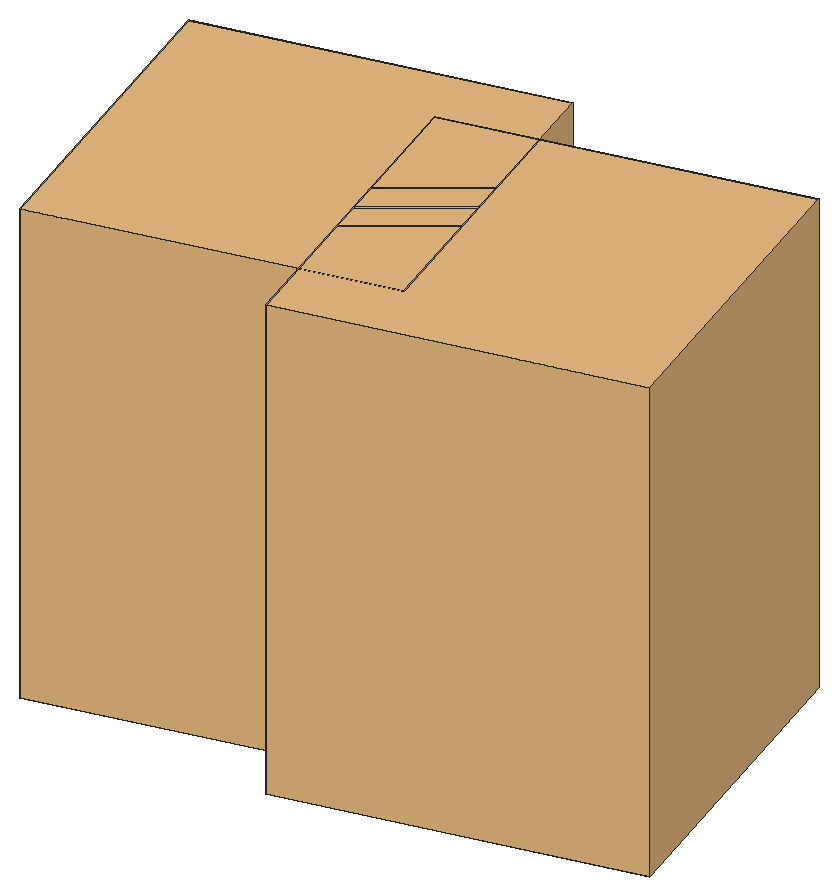
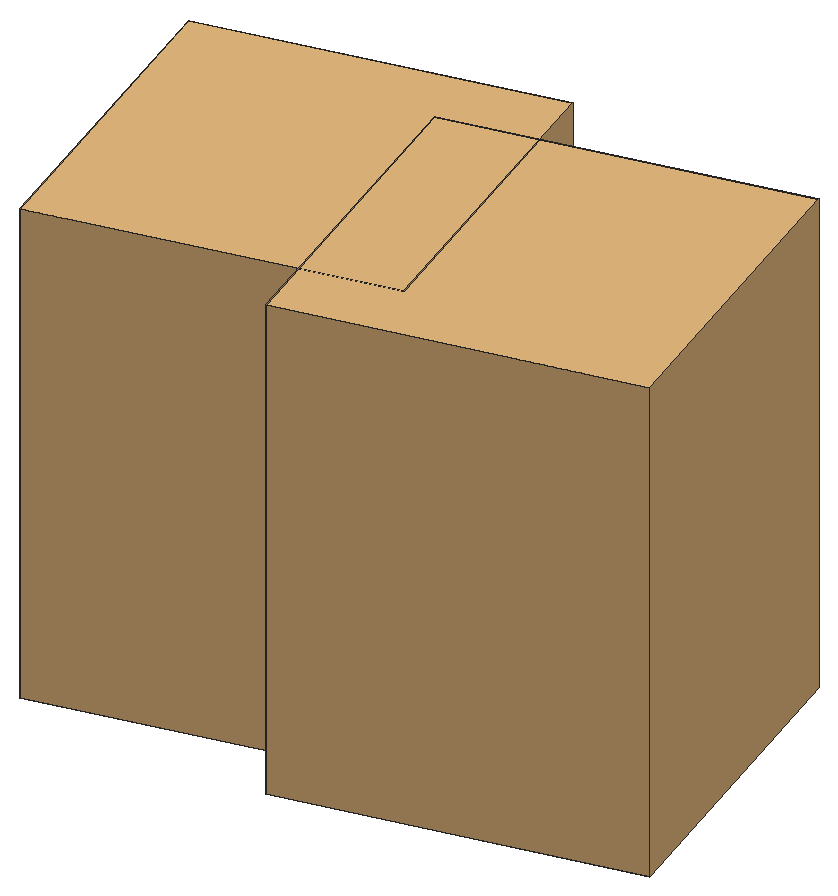
# SketchUp Ruby script. Lengths in inches.
U = 1.inch
M = Sketchup.active_model
def pt(a) = Geom::Point3d.new(a.map { |v| v * U })
def face(e, loops, mat)
  f = e.add_face(loops[0].map { |a| pt(a) })
  loops[1..].each { |l| e.add_face(l.map { |a| pt(a) }).erase! }
  f.material = f.back_material = mat if mat
  f
end
# faces: each face lists its corners as indices into pts; further lists are holes
def faces(e, pts, list, mat = nil) = list.each { |f| face(e, (f[0].is_a?(Array) ? f : [f]).map { |l| l.map { |i| pts[i] } }, mat) }
# xy, xz, yz: faces in a plane at the given z, y or x. An outline is a flat list of corners, or four numbers for a rectangle; further outlines are holes
def ring(l) = l.size == 4 ? [[l[0], l[1]], [l[2], l[1]], [l[2], l[3]], [l[0], l[3]]] : l.each_slice(2).to_a
def flat(e, list, mat, &to3) = list.each { |f| face(e, (f[0].is_a?(Array) ? f : [f]).map { |l| ring(l).map { |u, v| to3.(u, v) } }, mat) }
def xy(e, z, list, mat = nil) = flat(e, list, mat) { |x, y| [x, y, z] }
def xz(e, y, list, mat = nil) = flat(e, list, mat) { |x, z| [x, y, z] }
def yz(e, x, list, mat = nil) = flat(e, list, mat) { |y, z| [x, y, z] }
def lines(e, pts, list) = list.each { |a, b| e.add_line(pt(pts[a]), pt(pts[b])) }
# prism: a flat outline (further loops are holes) pulled along v
def prism(e, loops, v, mat = nil)
  f = face(e, loops, mat); d = Geom::Vector3d.new(v.map { |x| x * U })
  f.pushpull(f.normal.samedirection?(d) ? d.length : -d.length)
end
def box(e, o, s, mat = nil) = prism(e, [[o, [o[0] + s[0], o[1], o[2]], [o[0] + s[0], o[1] + s[1], o[2]], [o[0], o[1] + s[1], o[2]]]], [0, 0, s[2]], mat)
def at(x, y, z, deg = 0) = Geom::Transformation.translation(pt([x, y, z])) * Geom::Transformation.rotation(ORIGIN, Z_AXIS, deg.degrees)
def axes(o, x, y, z) = Geom::Transformation.new([*x, 0, *y, 0, *z, 0, *pt(o).to_a, 1])
def part(name) = M.definitions.add(name)
# library, detail: a bought-in or finely detailed component or shape, given as its bounding box
def library(name, o, s) = part(name).tap { |d| box(d.entities, o, s) }
def detail(e, o, s) = box(e.add_group.entities, o, s)
def put(e, d, t, mat = nil) = e.add_instance(d, t).tap { |i| i.material = mat if mat }
def group(e, t, mat = nil) = e.add_group.tap { |g| g.transformation = t; g.material = mat if mat }.entities
root = M.entities
M.materials.add("Material82").color = [68, 110, 58]
M.materials.add("Material83").color = [48, 90, 38]
M.materials.add("Material84").color = [68, 110, 48]
M.materials.add("Material85").color = [48, 90, 48]
M.materials.add("Material86").color = [58, 110, 58]
M.materials.add("Material87").color = [58, 90, 38]
M.materials.add("Material88").color = [68, 100, 58]
M.materials.add("Material89").color = [48, 100, 38]
c1 = part("grass00")
p = [[-0.6875,0.15,0],[-0.56,0.08,5.52],[-0.04,0.03,2.76],[0.48,-0.02,0],[0.35,-0.02,5.52],[-0.1,-0.14,5.52],
  [-0.12,0.65,8.37],[-0.42,0.65,8.37]]
faces(c1.entities,p,[[0,1,2,3],[3,2,4],[1,5,2],[5,4,2],[1,6,5],[4,5,6],[7,6,1]])
c2 = part("Group16\#1")
put(c2.entities,c1,axes([1.44,-0.61,-0.01],[0.05352,0.12609,0],[-0.10704,0.04543,0.07239],[0.06664,-0.02828,0.11628]),"Material85")
put(c2.entities,c1,axes([0.76,-0.15,-0.01],[0.04676,0.24062,0],[-0.23162,0.04501,0.06642],[0.0652,-0.01267,0.23595]),"Material82")
put(c2.entities,c1,axes([0.79,0.01,-0.01],[-0.00606,0.34651,0],[-0.34381,-0.00602,0.0432],[0.04319,0.00076,0.34386]))
put(c2.entities,c1,axes([1,0.23,-0.01],[-0.07192,0.31144,0],[-0.28722,-0.06632,0.1236],[0.12043,0.02781,0.29478]),"Material84")
put(c2.entities,c1,axes([1.66,0.77,-0.01],[-0.13828,0.29651,0],[-0.21551,-0.1005,0.22471],[0.20365,0.09498,0.23779]),"Material89")
put(c2.entities,c1,axes([0.6875,0.52,-0.01],[-0.18126,0.24051,0],[-0.22746,-0.17142,0.09788],[0.07817,0.05891,0.28481]),"Material84")
put(c2.entities,c1,axes([0.68,0.78,-0.01],[-0.215,0.18688,0],[-0.12385,-0.14248,0.21334],[0.13995,0.16101,0.18878]),"Material82")
put(c2.entities,c1,axes([0.56,1,-0.01],[-0.13756,0.07624,0],[-0.06159,-0.11112,0.0927],[0.04494,0.08108,0.12705]),"Material84")
put(c2.entities,c1,axes([0.2,0.64,-0.01],[-0.23729,0.07254,0],[-0.05711,-0.18681,0.153],[0.04473,0.14632,0.19535]),"Material89")
put(c2.entities,c1,axes([0.0625,0.72,-0.01],[-0.28874,0.02525,0],[-0.02179,-0.24916,0.14647],[0.01276,0.14591,0.25012]),"Material82")
put(c2.entities,c1,axes([-0.08,0.62,-0.01],[-0.34089,-0.04187,0],[0.03255,-0.26504,0.216],[-0.02633,0.21439,0.26703]),"Material89")
put(c2.entities,c1,axes([-0.34,0.98,-0.01],[-0.14314,-0.0493,0],[0.04397,-0.12769,0.06843],[-0.02228,0.0647,0.13505]),"Material89")
put(c2.entities,c1,axes([-0.87,1.45,-0.01],[-0.23488,-0.14114,0],[0.13761,-0.22901,0.06087],[-0.03135,0.05217,0.26717]))
put(c2.entities,c1,axes([-0.72,0.77,-0.01],[-0.14208,-0.13251,0],[0.07209,-0.0773,0.16301],[-0.11118,0.11922,0.1057]),"Material89")
put(c2.entities,c1,axes([-0.62,0.43,-0.01],[-0.14845,-0.21203,0],[0.18654,-0.13061,0.12304],[-0.10079,0.07057,0.22772]),"Material82")
put(c2.entities,c1,axes([-0.68,0.29,-0.01],[-0.13639,-0.32136,0],[0.31723,-0.13464,0.05579],[-0.05136,0.0218,0.34462]),"Material83")
put(c2.entities,c1,axes([-0.64,0.125,-0.01],[-0.0458,-0.23569,0],[0.22124,-0.043,0.08276],[-0.08124,0.01579,0.22538]),"Material86")
put(c2.entities,c1,axes([-1.6,-0.03,-0.01],[0.00576,-0.32897,0],[0.27526,0.00482,0.18018],[-0.18015,-0.00315,0.2753]),"Material84")
put(c2.entities,c1,axes([-1.36,-0.31,-0.01],[0.05718,-0.24765,0],[0.18172,0.04196,0.17267],[-0.16825,-0.03885,0.1865]),"Material89")
put(c2.entities,c1,axes([-1.54,-0.72,-0.01],[0.06537,-0.14017,0],[0.13555,0.06321,0.03939],[-0.0357,-0.01665,0.14956]))
put(c2.entities,c1,axes([-1.19,-0.9,-0.01],[0.09597,-0.12735,0],[0.11214,0.08451,0.07557],[-0.06035,-0.04548,0.14042]),"Material88")
put(c2.entities,c1,axes([-0.47,-0.54,-0.01],[0.11588,-0.10072,0],[0.0618,0.0711,0.12124],[-0.07953,-0.0915,0.0942]))
put(c2.entities,c1,axes([-0.47,-0.84,-0.01],[0.11927,-0.0661,0],[0.06603,0.11913,0.00646],[-0.00313,-0.00565,0.13621]),"Material84")
put(c2.entities,c1,axes([-0.38,-1.24,-0.01],[0.28037,-0.08571,0],[0.0618,0.20215,0.20315],[-0.05939,-0.19428,0.21139]),"Material88")
put(c2.entities,c1,axes([-0.06,-0.66,-0.01],[0.22719,-0.01987,0],[0.01247,0.14255,0.17758],[-0.01547,-0.17691,0.1431]),"Material87")
put(c2.entities,c1,axes([0.11,-0.89,-0.01],[0.14882,0.01828,0],[-0.01058,0.08611,0.12229],[0.01491,-0.12138,0.08676]),"Material85")
put(c2.entities,c1,axes([0.25,-0.72,-0.01],[0.20481,0.07053,0],[-0.06206,0.18022,0.10291],[0.03351,-0.0973,0.1906]),"Material85")
put(c2.entities,c1,axes([0.85,-1.42,-0.01],[0.16481,0.09904,0],[-0.09472,0.15762,0.05616],[0.02893,-0.04814,0.18389]),"Material84")
put(c2.entities,c1,axes([1.01,-1.09,-0.01],[0.21858,0.20385,0],[-0.17495,0.1876,0.15339],[0.10462,-0.11218,0.25652]),"Material89")
put(c2.entities,c1,axes([1.01,-0.71,-0.01],[0.08733,0.12473,0],[-0.06445,0.04512,0.13037],[0.1068,-0.07477,0.07867]),"Material85")
c3 = part("Group15\#1")
put(c3.entities,c2,at(0,0,0))
c4 = part("3darcstudiotree_grass00\#1")
put(c4.entities,c3,at(0,0,0))
c5 = library("Palm tree",[-4.09,-4.52,0],[193.52,193.51,258.93])
c6 = part("Palm+Tree")
put(c6.entities,c5,at(25.51,-21.81,0,15))
c7 = library("Group\#612",[0,0,0],[32.91,53.52,103.45])
put(root,c4,axes([1856.3125,966.58,-29.74],[3.38368,1.04745,0],[-2.27938,1.14521,-0.02005],[-0.08327,0.04184,1.86077]))
put(root,c4,axes([1858.36,994.28,-29.74],[0.01113,-1.45353,0],[4.54919,0.00542,-0.03692],[0.17089,0.0002,1.57831]))
put(root,c4,axes([1858.7,972.38,-29.74],[-1.2969,-1.20265,0],[3.80092,-0.63749,-0.01791],[0.10113,-0.01696,1.89984]))
put(root,c4,axes([1858.8,950.74,-29.74],[0.25593,-1.38573,0],[3.33259,0.09573,-0.00937],[0.07232,0.00208,1.93766]))
put(root,c4,axes([1858.69,946.16,-29.74],[-3.13946,0.49629,0],[-1.50487,-1.48058,-0.04281],[-0.09532,-0.09378,1.81418]))
put(root,c4,axes([1858.58,988.9,-29.74],[3.11316,-1.08854,0],[2.76667,1.23063,-0.03392],[0.0954,0.04244,1.32537]))
put(root,c4,axes([1859.6875,957.3,-29.74],[-3.90762,0.14516,0],[-0.37668,-1.57704,-0.0202],[-0.01231,-0.05153,1.95637]))
put(root,c4,axes([1858.54,941.52,-29.74],[3.63772,-0.04618,0],[0.1059,1.29755,-0.04101],[0.00733,0.08987,1.37186]))
put(root,c4,axes([1858.61,996.94,-29.74],[0.13497,1.53866,0],[-3.75353,0.05121,-0.02489],[-0.17047,0.00233,1.9295]))
put(root,c4,axes([1859.17,992.46,-29.74],[-2.50392,0.92561,0],[-3.00944,-1.26617,-0.02311],[-0.06646,-0.02796,1.38694]))
put(root,c4,axes([1860.33,985.73,-29.74],[-4.13167,0.24366,0],[-0.69238,-1.82599,-0.06496],[-0.05165,-0.1362,1.88637]))
put(root,c4,axes([1859.52,968.625,-29.74],[-1.70819,1.11812,0],[-3.96876,-0.943,-0.04504],[-0.21667,-0.05148,1.9506]))
put(root,c4,axes([1859.7,977.74,-29.74],[3.79912,-1.05543,0],[2.19489,1.22878,-0.03692],[0.13668,0.07652,1.83631]))
put(root,c4,axes([1859.58,943.99,-29.74],[3.28657,0.21022,0],[-0.53923,1.31117,-0.01255],[-0.01302,0.03166,1.63564]))
put(root,c4,axes([1860.18,983.93,-29.74],[-2.37455,1.29783,0],[-2.73236,-0.77752,-0.00844],[-0.03827,-0.01089,1.41311]))
put(root,c4,axes([1859.5,974.99,-29.74],[2.3712,1.21069,0],[-3.58151,1.09097,-0.04605],[-0.15475,0.04714,1.44046]))
put(root,c4,axes([1860.73,960.11,-29.74],[1.66455,-1.14728,0],[3.31311,0.74761,-0.04415],[0.26641,0.06012,1.98924]))
put(root,c4,axes([1861.84,990.33,-29.74],[-0.63027,-1.58552,0],[4.65732,-0.28794,-0.06318],[0.24644,-0.01524,1.39517]))
put(root,c4,axes([1860.29,961.55,-29.74],[2.52471,1.58546,0],[-3.52346,0.87265,-0.052],[-0.25077,0.06211,1.7759]))
put(root,c4,axes([1861.07,982.34,-29.74],[3.33412,-1.28398,0],[2.96352,1.19685,-0.04175],[0.14903,0.06019,1.62422]))
put(root,c4,axes([1860.47,978.86,-29.74],[3.98735,0.11869,0],[-0.3473,1.81468,-0.00004],[-0.00002,0.00009,1.93334]))
put(root,c4,axes([1862.11,953.3125,-29.74],[-2.08457,-1.53905,0],[3.84719,-0.81044,-0.05822],[0.30315,-0.06386,1.92982]))
put(root,c4,axes([1861.24,970.21,-29.74],[0.24653,1.78059,0],[-4.18646,0.09015,-0.05861],[-0.36644,0.00789,1.96776]))
put(root,c4,axes([1860.75,964.86,-29.74],[4.09909,0.70116,0],[-1.55013,1.40946,-0.01845],[-0.03388,0.03081,1.34771]))
put(root,c4,axes([1860.79,940.48,-29.74],[1.95248,1.61036,0],[-3.842,0.72449,-0.01048],[-0.04175,0.00787,1.40926]))
put(root,c4,axes([1861.11,955.24,-29.74],[3.93599,0.37319,0],[-1.10472,1.81211,-0.03506],[-0.03066,0.05029,1.32515]))
put(root,c4,axes([1861.76,948.9,-29.74],[3.76504,-0.34797,0],[1.07827,1.81452,-0.02268],[0.0226,0.03802,1.5468]))
put(root,c4,axes([1861.75,965.91,-29.74],[-0.03028,1.81071,0],[-4.52004,-0.01176,-0.01347],[-0.05788,-0.00015,1.45625]))
put(root,c4,axes([1863.97,947.37,-29.74],[2.88127,-0.83898,0],[2.47269,1.32072,-0.02283],[0.06307,0.03369,1.4512]))
put(root,c4,axes([1864.89,952.36,-29.74],[-1.69688,-1.72936,0],[4.23511,-0.64631,-0.05475],[0.2829,-0.04317,1.88574]))
put(root,c4,axes([1863.97,944.48,-29.74],[3.22121,-0.88629,0],[2.07064,1.17047,-0.00731],[0.02777,0.0157,1.80073]))
put(root,c4,axes([1865.1,994.51,-29.74],[-1.90792,-1.42621,0],[3.47826,-0.72369,-0.03938],[0.16408,-0.03414,1.38871]))
put(root,c4,axes([1864.16,981.1,-29.74],[3.56261,-0.94567,0],[1.87037,1.0959,-0.0013],[0.00431,0.00253,1.49257]))
put(root,c4,axes([1864.0625,955.86,-29.74],[-1.05565,1.36177,0],[-3.91341,-0.47183,-0.0271],[-0.14616,-0.01762,1.72974]))
put(root,c4,axes([1865.36,948.53,-29.74],[-4.0685,0.50795,0],[-1.17773,-1.46714,-0.03323],[-0.06082,-0.07576,1.77353]))
put(root,c4,axes([1864.42,941.89,-29.74],[4.25936,0.17724,0],[-0.36955,1.38123,-0.03171],[-0.02162,0.08082,1.71518]))
put(root,c4,axes([1866.03,958.15,-29.74],[0.20903,-1.7077,0],[3.89534,0.07416,-0.00402],[0.01821,0.00035,1.3243]))
put(root,c4,axes([1866.13,964.27,-29.74],[-3.49989,-0.62042,0],[1.34924,-1.18377,-0.02079],[0.0557,-0.04887,1.61237]))
put(root,c4,axes([1865.39,966.43,-29.74],[-2.24971,1.27376,0],[-2.901,-0.79689,-0.01437],[-0.08541,-0.02346,1.91898]))
put(root,c4,axes([1866.29,988.83,-29.74],[-2.13915,-1.27276,0],[3.26215,-0.85272,-0.05028],[0.27845,-0.07279,1.94898]))
put(root,c4,axes([1865.16,992.79,-29.74],[4.02195,-0.32221,0],[0.68718,1.33408,-0.00331],[0.00405,0.00786,1.58887]))
put(root,c4,axes([1864.66,979.09,-29.74],[4.32701,0.55712,0],[-1.36775,1.65217,-0.00124],[-0.00192,0.00232,1.65228]))
put(root,c4,axes([1865.85,986.48,-29.74],[-1.63539,1.16071,0],[-3.40916,-0.74706,-0.05151],[-0.29339,-0.06429,1.90487]))
put(root,c4,axes([1865.06,983.57,-29.74],[1.01762,1.37596,0],[-4.26505,0.49058,-0.00405],[-0.01582,0.00182,1.35389]))
put(root,c4,axes([1867.35,975.45,-29.74],[-3.3697,-1.02042,0],[2.44227,-1.25434,-0.00705],[0.02625,-0.01348,1.8369]))
put(root,c4,axes([1866.49,977.03,-29.74],[2.02024,-1.18426,0],[3.76291,0.99837,-0.06298],[0.20491,0.05437,1.33293]))
put(root,c4,axes([1865.71,940.4,-29.74],[4.3094,-0.16311,0],[0.42718,1.75528,-0.01064],[0.00539,0.02213,1.77558]))
put(root,c4,axes([1867.47,990.66,-29.74],[-2.95002,-1.42448,0],[3.56758,-1.14909,-0.03335],[0.13906,-0.04479,1.85855]))
put(root,c4,axes([1866.9,971.42,-29.74],[0.35372,-1.85816,0],[4.64402,0.13749,-0.06273],[0.35272,0.01044,1.9684]))
put(root,c4,axes([1866.49,950.38,-29.74],[-1.74852,1.13217,0],[-3.21789,-0.77293,-0.03041],[-0.12145,-0.02917,1.3205]))
put(root,c4,axes([1867.8125,969.18,-29.74],[-1.80602,-1.23313,0],[3.1704,-0.72217,-0.00817],[0.04009,-0.00913,1.55447]))
put(root,c4,axes([1867.05,972.1,-29.74],[3.72507,-0.62439,0],[1.73357,1.60854,-0.00549],[0.00931,0.00864,1.44062]))
put(root,c4,axes([1867.05,960.3,-29.74],[3.99736,-0.43263,0],[1.22188,1.75587,-0.05143],[0.05673,0.08152,1.44218]))
put(root,c4,axes([1867.01,962.125,-29.74],[-0.70731,1.48216,0],[-4.42453,-0.32839,-0.01956],[-0.1033,-0.00767,1.8138]))
put(root,c4,axes([1869.49,958,-29.74],[-4.33089,0.41445,0],[-1.11243,-1.80796,-0.06662],[-0.06204,-0.10083,1.39642]))
put(root,c4,axes([1870.375,948.14,-29.74],[-3.26976,-0.5137,0],[1.67175,-1.65498,-0.00121],[0.00254,-0.00252,1.92636]))
put(root,c4,axes([1869.61,992.46,-29.74],[1.4091,-1.17417,0],[3.00858,0.56155,-0.04441],[0.31581,0.05895,1.96303]))
put(root,c4,axes([1870.35,988.18,-29.74],[-0.33318,-1.39627,0],[3.47077,-0.12881,-0.04952],[0.2452,-0.0091,1.29958]))
put(root,c4,axes([1870.46,983.83,-29.74],[-3.53744,1.16554,0],[-2.5606,-1.20869,-0.03098],[-0.10582,-0.04995,1.59479]))
put(root,c4,axes([1871.08,996.27,-29.74],[-3.84526,-0.22431,0],[0.50015,-1.33348,-0.00812],[0.00644,-0.01718,1.3892]))
put(root,c4,axes([1870.6,978.95,-29.74],[-3.00421,0.76942,0],[-2.15411,-1.30812,-0.04277],[-0.14646,-0.08894,1.86401]))
put(root,c4,axes([1870.06,950.6,-29.74],[-0.58592,1.57945,0],[-3.44253,-0.19862,-0.02144],[-0.15876,-0.00916,1.9513]))
put(root,c4,axes([1870.57,971.43,-29.74],[-3.04736,0.88871,0],[-2.40783,-1.28411,-0.01371],[-0.03527,-0.01881,1.31321]))
put(root,c4,axes([1870.0625,990.875,-29.74],[3.34176,-0.01383,0],[0.04057,1.52455,-0.01029],[0.00052,0.01945,1.389]))
put(root,c4,axes([1871.1875,955.2,-29.74],[1.49416,-1.17809,0],[3.55261,0.70077,-0.01805],[0.08589,0.01694,1.58457]))
put(root,c4,axes([1870.31,977.41,-29.74],[3.91979,-0.74164,0],[1.60866,1.32236,-0.04597],[0.11253,0.0925,1.57738]))
put(root,c4,axes([1870.49,974.67,-29.74],[-2.1963,1.32957,0],[-3.96988,-1.01993,-0.00953],[-0.0332,-0.00853,1.47621]))
put(root,c4,axes([1871.74,994.88,-29.74],[0.96851,-1.36822,0],[3.89034,0.4283,-0.00232],[0.01298,0.00143,1.76107]))
put(root,c4,axes([1870.74,981.86,-29.74],[3.27047,-0.2692,0],[0.72961,1.37861,-0.04941],[0.05481,0.10356,1.4533]))
put(root,c4,axes([1871.97,964.88,-29.74],[2.10515,-1.21949,0],[3.30844,0.88826,-0.01892],[0.09087,0.0244,1.74337]))
put(root,c4,axes([1871.85,943.72,-29.74],[-2.16702,1.28274,0],[-3.03597,-0.79769,-0.03773],[-0.16249,-0.04269,1.41517]))
put(root,c4,axes([1871.08,985.74,-29.74],[4.03817,0.43694,0],[-1.08149,1.5545,-0.02738],[-0.04454,0.06402,1.88342]))
put(root,c4,axes([1871.63,972.08,-29.74],[4.33985,-0.71517,0],[1.81915,1.7169,-0.05614],[0.0962,0.09079,1.57175]))
put(root,c4,axes([1872.65,960.42,-29.74],[1.94166,-1.68054,0],[3.68889,0.66287,-0.02827],[0.1643,0.02952,1.94019]))
put(root,c4,axes([1871.95,966.31,-29.74],[0.75441,1.71197,0],[-3.26624,0.22386,-0.03272],[-0.2394,0.01641,1.8454]))
put(root,c4,axes([1871.6875,968.55,-29.74],[2.94946,0.97112,0],[-2.79078,1.31828,-0.05497],[-0.191,0.09022,1.76958]))
put(root,c4,axes([1871.66,961.14,-29.74],[2.19107,1.06462,0],[-2.74426,0.87841,-0.00448],[-0.02021,0.00647,1.5389]))
put(root,c4,axes([1872.82,953.46,-29.74],[2.33071,-1.20912,0],[3.74929,1.12403,-0.05929],[0.20074,0.06018,1.50135]))
put(root,c4,axes([1872.5625,942.1875,-29.74],[-0.50717,1.45325,0],[-4.1597,-0.22578,-0.0385],[-0.18859,-0.01024,1.55608]))
put(root,c4,axes([1872.95,946.87,-29.74],[4.27397,-0.60338,0],[1.4489,1.5962,-0.05713],[0.08848,0.09748,1.48067]))
put(root,c4,axes([1875,985.39,-29.74],[-2.9256,-1.47399,0],[3.63184,-1.12114,-0.01534],[0.06015,-0.01857,1.72134]))
put(root,c4,axes([1874.78,970.86,-29.74],[-4.1987,0.12334,0],[-0.25997,-1.37638,-0.0204],[-0.0079,-0.04182,1.3669]))
put(root,c4,axes([1875.15,990.07,-29.74],[-4.00085,-0.57986,0],[1.27846,-1.37193,-0.00277],[0.00474,-0.00509,1.38049]))
put(root,c4,axes([1875.67,973.33,-29.74],[-3.39001,-0.81782,0],[2.4179,-1.55881,-0.03935],[0.08518,-0.05492,1.44076]))
put(root,c4,axes([1874.99,946.19,-29.74],[3.84648,-0.75898,0],[1.52103,1.1989,-0.01525],[0.0428,0.03373,1.59832]))
put(root,c4,axes([1875.625,979.42,-29.74],[2.20697,-0.9726,0],[2.75858,0.97355,-0.01984],[0.09708,0.03426,1.82222]))
put(root,c4,axes([1875.44,974.45,-29.74],[0.68368,1.71904,0],[-3.38759,0.20954,-0.03929],[-0.29518,0.01826,1.95437]))
put(root,c4,axes([1876.92,981.53,-29.74],[-2.04632,-1.05436,0],[3.10393,-0.93693,-0.02737],[0.09658,-0.02915,1.30175]))
put(root,c4,axes([1875.84,968.07,-29.74],[-0.28903,1.73584,0],[-3.34699,-0.08668,-0.03425],[-0.21957,-0.00569,1.61497]))
put(root,c4,axes([1876.68,988.55,-29.74],[1.71259,-1.30416,0],[3.53393,0.72176,-0.01075],[0.04765,0.00973,1.48923]))
put(root,c4,axes([1876.95,954.71,-29.74],[-3.772,0.03773,0],[-0.10384,-1.61464,-0.00196],[-0.00024,-0.00377,1.49745]))
put(root,c4,axes([1876.29,949.1,-29.74],[-2.36342,1.1502,0],[-3.36153,-1.07427,-0.04128],[-0.15124,-0.04833,1.52936]))
put(root,c4,axes([1875.87,953.5,-29.74],[4.05183,0.05747,0],[-0.14664,1.60785,-0.02702],[-0.00634,0.06949,1.99535]))
put(root,c4,axes([1876.77,997.43,-29.74],[2.29885,-0.96399,0],[2.83055,1.04983,-0.02136],[0.08662,0.03213,1.62144]))
put(root,c4,axes([1877.5,951.28,-29.74],[-4.17405,-0.19289,0],[0.40333,-1.35747,-0.00847],[0.00693,-0.02334,1.82708]))
put(root,c4,axes([1876.45,977.7,-29.74],[1.65421,1.20964,0],[-3.07102,0.65317,-0.03445],[-0.21317,0.04534,1.83855]))
put(root,c4,axes([1878.15,945.24,-29.74],[-2.90823,-0.76432,0],[2.41266,-1.42777,-0.04785],[0.14851,-0.08788,1.82518]))
put(root,c4,axes([1877.18,964.84,-29.74],[-1.04428,1.44728,0],[-3.25699,-0.36551,-0.00052],[-0.00331,-0.00037,1.67384]))
put(root,c4,axes([1877.31,965.93,-29.74],[3.83018,0.17914,0],[-0.49889,1.65896,-0.05841],[-0.02825,0.09394,1.30397]))
put(root,c4,axes([1878.83,959.08,-29.74],[-3.60335,-0.2844,0],[0.69529,-1.3701,-0.00178],[0.00231,-0.00455,1.75352]))
put(root,c4,axes([1878.28,983.46,-29.74],[-2.93874,0.89671,0],[-2.33959,-1.1925,-0.04163],[-0.12402,-0.06321,1.39503]))
put(root,c4,axes([1877.42,992.11,-29.74],[2.61631,0.861,0],[-2.17217,1.02658,-0.00812],[-0.03307,0.01563,1.6158]))
put(root,c4,axes([1877.38,957.84,-29.74],[2.19518,1.25426,0],[-3.21279,0.87453,-0.02215],[-0.10628,0.02893,1.70619]))
put(root,c4,axes([1878.05,941.48,-29.74],[0.43339,1.54675,0],[-3.36238,0.14653,-0.03685],[-0.25104,0.01094,1.73767]))
put(root,c4,axes([1877.68,993.9375,-29.74],[3.82301,1.06562,0],[-2.5922,1.44638,-0.0169],[-0.04207,0.02347,1.45184]))
put(root,c4,axes([1878.625,961.87,-29.74],[3.73956,-0.25134,0],[0.58802,1.36068,-0.03176],[0.03776,0.08738,1.85682]))
put(root,c4,axes([1880.5,954.85,-29.74],[-2.3605,-1.50274,0],[2.8114,-0.68684,-0.00146],[0.00663,-0.00162,1.32424]))
put(root,c4,axes([1880.45,949.35,-29.74],[3.76532,-0.82989,0],[2.11238,1.49062,-0.04605],[0.09606,0.06778,1.38783]))
put(root,c4,axes([1881.72,946.32,-29.74],[-2.75712,-0.97177,0],[2.36987,-1.04575,-0.04195],[0.16334,-0.07208,1.55746]))
put(root,c4,axes([1880.29,992.35,-29.74],[1.13904,1.65719,0],[-4.07352,0.43546,-0.03421],[-0.20227,0.02162,1.93796]))
put(root,c4,axes([1882.29,962.58,-29.74],[-1.0442,-1.68413,0],[4.42012,-0.42624,-0.03172],[0.12352,-0.01191,1.36741]))
put(root,c4,axes([1882.44,942.29,-29.74],[-2.93582,-0.70247,0],[2.08855,-1.35755,-0.00574],[0.01328,-0.00863,1.3472]))
put(root,c4,axes([1882.47,971.36,-29.74],[-2.87675,-1.09055,0],[2.6601,-1.09136,-0.02949],[0.13969,-0.05731,1.96656]))
put(root,c4,axes([1882.61,976.82,-29.74],[-2.96111,-1.38906,0],[2.74036,-0.90856,-0.02964],[0.13819,-0.04582,1.63454]))
put(root,c4,axes([1881.01,960.22,-29.74],[2.75422,1.28702,0],[-2.68657,0.89417,-0.05003],[-0.26479,0.08813,1.82479]))
put(root,c4,axes([1881.18,966.43,-29.74],[2.36808,1.36159,0],[-2.95794,0.80011,-0.03781],[-0.20263,0.05481,1.74723]))
put(root,c4,axes([1881.24,994.65,-29.74],[4.47082,0.11069,0],[-0.26321,1.65346,-0.04601],[-0.01202,0.07548,1.31249]))
put(root,c4,axes([1881.88,975.17,-29.74],[-2.49032,1.32428,0],[-3.19574,-0.93467,-0.0152],[-0.05407,-0.01581,1.3203]))
put(root,c4,axes([1881.33,967.68,-29.74],[1.04539,1.48143,0],[-4.29845,0.47176,-0.02844],[-0.1492,0.01637,1.82107]))
put(root,c4,axes([1882.1,988.1875,-29.74],[-2.32252,1.56487,0],[-3.68383,-0.85034,-0.03733],[-0.14959,-0.03453,1.48568]))
put(root,c4,axes([1881.49,983.05,-29.74],[2.07418,1.09295,0],[-3.13936,0.92662,-0.0157],[-0.06877,0.0203,1.60759]))
put(root,c4,axes([1882.19,963.48,-29.74],[3.63146,-0.94763,0],[2.16895,1.29272,-0.03005],[0.10609,0.06323,1.88475]))
put(root,c4,axes([1881.79,973.6,-29.74],[0.90968,1.754,0],[-3.81846,0.30801,-0.01369],[-0.06439,0.00519,1.40267]))
put(root,c4,axes([1882.38,944.52,-29.74],[0.278,1.64734,0],[-3.85699,0.10123,-0.01024],[-0.06423,0.00169,1.82096]))
put(root,c4,axes([1882.88,980.76,-29.74],[-1.2304,1.69187,0],[-3.83777,-0.43408,-0.02925],[-0.12783,-0.01446,1.36051]))
put(root,c4,axes([1882.55,986.38,-29.74],[2.50159,1.07866,0],[-2.96417,1.06917,-0.03451],[-0.16033,0.05783,1.89576]))
put(root,c4,axes([1882.69,990.76,-29.74],[3.85299,0.72056,0],[-1.4234,1.18377,-0.0026],[-0.00811,0.00675,1.81639]))
put(root,c4,axes([1884.25,953.26,-29.74],[-3.94572,0.20967,0],[-0.54102,-1.58348,-0.01091],[-0.00895,-0.02619,1.8656]))
put(root,c4,axes([1882.89,950.24,-29.74],[4.67805,0.10708,0],[-0.2535,1.72242,-0.0212],[-0.00736,0.05004,1.96575]))
put(root,c4,axes([1883.18,979,-29.74],[3.89819,0.51903,0],[-1.48599,1.73579,-0.0473],[-0.0826,0.09649,1.90097]))
put(root,c4,axes([1883.24,997.3,-29.74],[3.72345,0.43237,0],[-1.05501,1.41306,-0.01058],[-0.0164,0.02196,1.53588]))
put(root,c4,axes([1883.41,957.49,-29.74],[3.62609,0.38691,0],[-0.94095,1.37154,-0.04799],[-0.07441,0.10847,1.60328]))
put(root,c4,axes([1886.5,946.9,-29.74],[-2.74827,-0.90606,0],[2.5057,-1.18207,-0.04185],[0.15974,-0.07536,1.7425]))
put(root,c4,axes([1886.78,978.92,-29.74],[-2.21298,-1.13198,0],[3.27865,-0.99688,-0.03514],[0.15829,-0.04813,1.76492]))
put(root,c4,axes([1886.72,990.26,-29.74],[1.56077,-1.21628,0],[3.51485,0.70149,-0.00728],[0.02929,0.00585,1.33141]))
put(root,c4,axes([1886.2,992.375,-29.74],[-1.38329,1.54062,0],[-3.20389,-0.44741,-0.04758],[-0.27737,-0.03873,1.57537]))
put(root,c4,axes([1887.26,951.05,-29.74],[-4.11808,-0.53305,0],[1.24091,-1.491,-0.0393],[0.07027,-0.08443,1.71017]))
put(root,c4,axes([1886.83,982.05,-29.74],[-3.99092,0.85507,0],[-1.6879,-1.22527,-0.00649],[-0.01661,-0.01206,1.42064]))
put(root,c4,axes([1886.18,994.9,-29.74],[-0.13254,1.67215,0],[-3.60359,-0.04442,-0.04056],[-0.20717,-0.00255,1.38085]))
put(root,c4,axes([1887.03,961.12,-29.74],[-1.8566,1.22673,0],[-3.23788,-0.76215,-0.0186],[-0.08298,-0.01953,1.46845]))
put(root,c4,axes([1887.21,972.03,-29.74],[3.63516,-0.37062,0],[1.04175,1.58916,-0.04398],[0.06662,0.10163,1.88821]))
put(root,c4,axes([1887.15,942.59,-29.74],[4.38242,0.53414,0],[-1.34963,1.72221,-0.04987],[-0.06942,0.08859,1.61513]))
put(root,c6,at(1831.54,891.52,-29.74))
put(root,c7,axes([1999.23,894.49,-29.74],[1.13014,0.75656,0],[-0.75656,1.13014,0],[0,0,1.36]))
put(root,c6,at(1976.92,891.52,-29.74))
